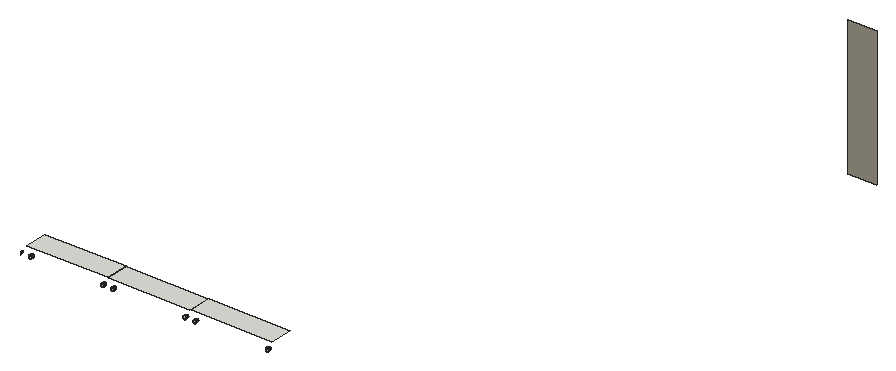
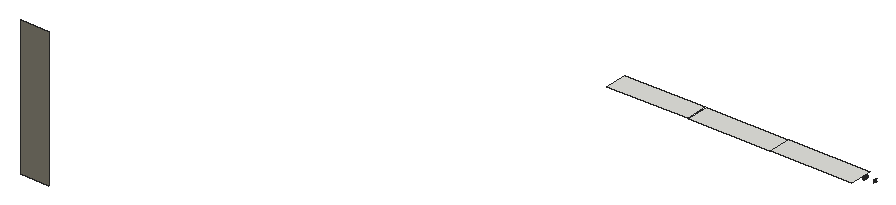
# SketchUp Ruby script. Lengths in inches.
U = 1.inch
M = Sketchup.active_model
def pt(a) = Geom::Point3d.new(a.map { |v| v * U })
def face(e, loops, mat)
  f = e.add_face(loops[0].map { |a| pt(a) })
  loops[1..].each { |l| e.add_face(l.map { |a| pt(a) }).erase! }
  f.material = f.back_material = mat if mat
  f
end
# faces: each face lists its corners as indices into pts; further lists are holes
def faces(e, pts, list, mat = nil) = list.each { |f| face(e, (f[0].is_a?(Array) ? f : [f]).map { |l| l.map { |i| pts[i] } }, mat) }
# xy, xz, yz: faces in a plane at the given z, y or x. An outline is a flat list of corners, or four numbers for a rectangle; further outlines are holes
def ring(l) = l.size == 4 ? [[l[0], l[1]], [l[2], l[1]], [l[2], l[3]], [l[0], l[3]]] : l.each_slice(2).to_a
def flat(e, list, mat, &to3) = list.each { |f| face(e, (f[0].is_a?(Array) ? f : [f]).map { |l| ring(l).map { |u, v| to3.(u, v) } }, mat) }
def xy(e, z, list, mat = nil) = flat(e, list, mat) { |x, y| [x, y, z] }
def xz(e, y, list, mat = nil) = flat(e, list, mat) { |x, z| [x, y, z] }
def yz(e, x, list, mat = nil) = flat(e, list, mat) { |y, z| [x, y, z] }
def lines(e, pts, list) = list.each { |a, b| e.add_line(pt(pts[a]), pt(pts[b])) }
# prism: a flat outline (further loops are holes) pulled along v
def prism(e, loops, v, mat = nil)
  f = face(e, loops, mat); d = Geom::Vector3d.new(v.map { |x| x * U })
  f.pushpull(f.normal.samedirection?(d) ? d.length : -d.length)
end
def box(e, o, s, mat = nil) = prism(e, [[o, [o[0] + s[0], o[1], o[2]], [o[0] + s[0], o[1] + s[1], o[2]], [o[0], o[1] + s[1], o[2]]]], [0, 0, s[2]], mat)
def at(x, y, z, deg = 0) = Geom::Transformation.translation(pt([x, y, z])) * Geom::Transformation.rotation(ORIGIN, Z_AXIS, deg.degrees)
def axes(o, x, y, z) = Geom::Transformation.new([*x, 0, *y, 0, *z, 0, *pt(o).to_a, 1])
def part(name) = M.definitions.add(name)
# library, detail: a bought-in or finely detailed component or shape, given as its bounding box
def library(name, o, s) = part(name).tap { |d| box(d.entities, o, s) }
def detail(e, o, s) = box(e.add_group.entities, o, s)
def put(e, d, t, mat = nil) = e.add_instance(d, t).tap { |i| i.material = mat if mat }
def group(e, t, mat = nil) = e.add_group.tap { |g| g.transformation = t; g.material = mat if mat }.entities
root = M.entities
M.materials.add("[Concrete Tile]").color = [155, 150, 134]
xy(root,138.0625,[[1787.65,801.78,1844.77,817.6],[1845.83,801.78,1902.82,817.6],[1904.13,801.78,1960.87,817.6]])
xz(root,799.91,[[1791.54,131.88,1791.83,131.92,1792.1,132.03,1792.34,132.21,1792.51,132.44,1792.63,132.71,1792.67,133,1792.63,133.29,1792.51,133.57,1792.34,133.8,1792.1,133.98,1791.83,134.09,1791.54,134.13,1791.25,134.09,1790.98,133.98,1790.74,133.8,1790.57,133.57,1790.45,133.29,1790.42,133,1790.45,132.71,1790.57,132.44,1790.74,132.21,1790.98,132.03,1791.25,131.92],[1842.67,131.88,1842.96,131.92,1843.23,132.03,1843.46,132.21,1843.64,132.44,1843.75,132.71,1843.79,133,1843.75,133.29,1843.64,133.57,1843.46,133.8,1843.23,133.98,1842.96,134.09,1842.67,134.13,1842.375,134.09,1842.1,133.98,1841.87,133.8,1841.69,133.57,1841.58,133.29,1841.54,133,1841.58,132.71,1841.69,132.44,1841.87,132.21,1842.1,132.03,1842.375,131.92],[1849.72,131.88,1850.01,131.92,1850.28,132.03,1850.51,132.21,1850.69,132.44,1850.8,132.71,1850.84,133,1850.8,133.29,1850.69,133.57,1850.51,133.8,1850.28,133.98,1850.01,134.09,1849.72,134.13,1849.42,134.09,1849.15,133.98,1848.92,133.8,1848.74,133.57,1848.63,133.29,1848.59,133,1848.63,132.71,1848.74,132.44,1848.92,132.21,1849.15,132.03,1849.42,131.92],[1900.84,131.88,1901.13,131.92,1901.4,132.03,1901.64,132.21,1901.82,132.44,1901.93,132.71,1901.97,133,1901.93,133.29,1901.82,133.57,1901.64,133.8,1901.4,133.98,1901.13,134.09,1900.84,134.13,1900.55,134.09,1900.28,133.98,1900.05,133.8,1899.87,133.57,1899.75,133.29,1899.72,133,1899.75,132.71,1899.87,132.44,1900.05,132.21,1900.28,132.03,1900.55,131.92],[1908.02,131.88,1908.31,131.92,1908.58,132.03,1908.8125,132.21,1908.99,132.44,1909.1,132.71,1909.14,133,1909.1,133.29,1908.99,133.57,1908.8125,133.8,1908.58,133.98,1908.31,134.09,1908.02,134.13,1907.73,134.09,1907.45,133.98,1907.22,133.8,1907.04,133.57,1906.93,133.29,1906.89,133,1906.93,132.71,1907.04,132.44,1907.22,132.21,1907.45,132.03,1907.73,131.92],
  [1959.14,131.88,1959.43,131.92,1959.7,132.03,1959.9375,132.21,1960.12,132.44,1960.23,132.71,1960.27,133,1960.23,133.29,1960.12,133.57,1959.9375,133.8,1959.7,133.98,1959.43,134.09,1959.14,134.13,1958.85,134.09,1958.58,133.98,1958.35,133.8,1958.17,133.57,1958.06,133.29,1958.02,133,1958.06,132.71,1958.17,132.44,1958.35,132.21,1958.58,132.03,1958.85,131.92]])
xz(root,1122.97,[[2112.0625,156.5,2132.1875,254.125]],"[Concrete Tile]")
p = [[1790.98,801.78,132.03],[1791.25,801.78,131.92],[1791.25,799.91,131.92],[1790.98,799.91,132.03],[1791.54,801.78,131.88],[1791.54,799.91,131.88],
  [1791.83,801.78,131.92],[1791.83,799.91,131.92],[1792.1,801.78,132.03],[1792.1,799.91,132.03],[1842.1,801.78,132.03],[1842.375,801.78,131.92],
  [1842.375,799.91,131.92],[1842.1,799.91,132.03],[1842.67,801.78,131.88],[1842.67,799.91,131.88],[1842.96,801.78,131.92],[1842.96,799.91,131.92],
  [1843.23,801.78,132.03],[1843.23,799.91,132.03],[1849.15,801.78,132.03],[1849.42,801.78,131.92],[1849.42,799.91,131.92],[1849.15,799.91,132.03],
  [1849.72,801.78,131.88],[1849.72,799.91,131.88],[1850.01,801.78,131.92],[1850.01,799.91,131.92],[1850.28,801.78,132.03],[1850.28,799.91,132.03],
  [1900.28,801.78,132.03],[1900.55,801.78,131.92],[1900.55,799.91,131.92],[1900.28,799.91,132.03],[1900.84,801.78,131.88],[1900.84,799.91,131.88],
  [1901.13,801.78,131.92],[1901.13,799.91,131.92],[1901.4,801.78,132.03],[1901.4,799.91,132.03],[1907.45,801.78,132.03],[1907.73,801.78,131.92],
  [1907.73,799.91,131.92],[1907.45,799.91,132.03],[1908.02,801.78,131.88],[1908.02,799.91,131.88],[1908.31,801.78,131.92],[1908.31,799.91,131.92],
  [1908.58,801.78,132.03],[1908.58,799.91,132.03],[1958.58,801.78,132.03],[1958.85,801.78,131.92],[1958.85,799.91,131.92],[1958.58,799.91,132.03],
  [1959.14,801.78,131.88],[1959.14,799.91,131.88],[1959.43,801.78,131.92],[1959.43,799.91,131.92],[1959.7,801.78,132.03],[1959.7,799.91,132.03],
  [1790.74,801.78,132.21],[1790.74,799.91,132.21],[1792.34,801.78,132.21],[1792.34,799.91,132.21],[1841.87,801.78,132.21],[1841.87,799.91,132.21],
  [1843.46,801.78,132.21],[1843.46,799.91,132.21],[1848.92,801.78,132.21],[1848.92,799.91,132.21],[1850.51,801.78,132.21],[1850.51,799.91,132.21],
  [1900.05,801.78,132.21],[1900.05,799.91,132.21],[1901.64,801.78,132.21],[1901.64,799.91,132.21],[1907.22,801.78,132.21],[1907.22,799.91,132.21],
  [1908.8125,801.78,132.21],[1908.8125,799.91,132.21],[1958.35,801.78,132.21],[1958.35,799.91,132.21],[1959.9375,801.78,132.21],[1959.9375,799.91,132.21],
  [1784.47,801.78,132.21],[1784.65,801.78,132.44],[1784.65,799.91,132.44],[1784.47,799.91,132.21],[1790.57,801.78,132.44],[1790.57,799.91,132.44],
  [1792.51,801.78,132.44],[1792.51,799.91,132.44],[1841.69,801.78,132.44],[1841.69,799.91,132.44],[1843.64,801.78,132.44],[1843.64,799.91,132.44],
  [1848.74,801.78,132.44],[1848.74,799.91,132.44],[1850.69,801.78,132.44],[1850.69,799.91,132.44],[1899.87,801.78,132.44],[1899.87,799.91,132.44],
  [1901.82,801.78,132.44],[1901.82,799.91,132.44],[1907.04,801.78,132.44],[1907.04,799.91,132.44],[1908.99,801.78,132.44],[1908.99,799.91,132.44],
  [1958.17,801.78,132.44],[1958.17,799.91,132.44],[1960.12,801.78,132.44],[1960.12,799.91,132.44],[1784.76,801.78,132.71],[1784.76,799.91,132.71],
  [1790.45,801.78,132.71],[1790.45,799.91,132.71],[1792.63,801.78,132.71],[1792.63,799.91,132.71],[1841.58,801.78,132.71],[1841.58,799.91,132.71],
  [1843.75,801.78,132.71],[1843.75,799.91,132.71],[1848.63,801.78,132.71],[1848.63,799.91,132.71],[1850.8,801.78,132.71],[1850.8,799.91,132.71],
  [1899.75,801.78,132.71],[1899.75,799.91,132.71],[1901.93,801.78,132.71],[1901.93,799.91,132.71],[1906.93,801.78,132.71],[1906.93,799.91,132.71],
  [1909.1,801.78,132.71],[1909.1,799.91,132.71],[1958.06,801.78,132.71],[1958.06,799.91,132.71],[1960.23,801.78,132.71],[1960.23,799.91,132.71],
  [1784.8,801.78,133],[1784.8,799.91,133],[1790.42,801.78,133],[1790.42,799.91,133],[1792.67,801.78,133],[1792.67,799.91,133],
  [1841.54,801.78,133],[1841.54,799.91,133],[1843.79,801.78,133],[1843.79,799.91,133],[1848.59,801.78,133],[1848.59,799.91,133],
  [1850.84,801.78,133],[1850.84,799.91,133],[1899.72,801.78,133],[1899.72,799.91,133],[1901.97,801.78,133],[1901.97,799.91,133],
  [1906.89,801.78,133],[1906.89,799.91,133],[1909.14,801.78,133],[1909.14,799.91,133],[1958.02,801.78,133],[1958.02,799.91,133],
  [1960.27,801.78,133],[1960.27,799.91,133],[1784.76,801.78,133.29],[1784.76,799.91,133.29],[1790.45,801.78,133.29],[1790.45,799.91,133.29],
  [1792.63,801.78,133.29],[1792.63,799.91,133.29],[1841.58,801.78,133.29],[1841.58,799.91,133.29],[1843.75,801.78,133.29],[1843.75,799.91,133.29],
  [1848.63,801.78,133.29],[1848.63,799.91,133.29],[1850.8,801.78,133.29],[1850.8,799.91,133.29],[1899.75,801.78,133.29],[1899.75,799.91,133.29],
  [1901.93,801.78,133.29],[1901.93,799.91,133.29],[1906.93,801.78,133.29],[1906.93,799.91,133.29],[1909.1,801.78,133.29],[1909.1,799.91,133.29],
  [1958.06,801.78,133.29],[1958.06,799.91,133.29],[1960.23,801.78,133.29],[1960.23,799.91,133.29],[1784.65,801.78,133.57],[1784.65,799.91,133.57],
  [1790.57,801.78,133.57],[1790.57,799.91,133.57],[1792.51,801.78,133.57],[1792.51,799.91,133.57],[1841.69,801.78,133.57],[1841.69,799.91,133.57],
  [1843.64,801.78,133.57],[1843.64,799.91,133.57],[1848.74,801.78,133.57],[1848.74,799.91,133.57],[1850.69,801.78,133.57],[1850.69,799.91,133.57],
  [1899.87,801.78,133.57],[1899.87,799.91,133.57],[1901.82,801.78,133.57],[1901.82,799.91,133.57],[1907.04,801.78,133.57],[1907.04,799.91,133.57],
  [1908.99,801.78,133.57],[1908.99,799.91,133.57],[1958.17,801.78,133.57],[1958.17,799.91,133.57],[1960.12,801.78,133.57],[1960.12,799.91,133.57],
  [1784.47,801.78,133.8],[1784.47,799.91,133.8],[1790.74,801.78,133.8],[1790.74,799.91,133.8],[1792.34,801.78,133.8],[1792.34,799.91,133.8],
  [1841.87,801.78,133.8],[1841.87,799.91,133.8],[1843.46,801.78,133.8],[1843.46,799.91,133.8],[1848.92,801.78,133.8],[1848.92,799.91,133.8],
  [1850.51,801.78,133.8],[1850.51,799.91,133.8],[1900.05,801.78,133.8],[1900.05,799.91,133.8],[1901.64,801.78,133.8],[1901.64,799.91,133.8],
  [1907.22,801.78,133.8],[1907.22,799.91,133.8],[1908.8125,801.78,133.8],[1908.8125,799.91,133.8],[1958.35,801.78,133.8],[1958.35,799.91,133.8],
  [1959.9375,801.78,133.8],[1959.9375,799.91,133.8],[1790.98,801.78,133.98],[1790.98,799.91,133.98],[1792.1,801.78,133.98],[1792.1,799.91,133.98],
  [1842.1,801.78,133.98],[1842.1,799.91,133.98],[1843.23,801.78,133.98],[1843.23,799.91,133.98],[1849.15,801.78,133.98],[1849.15,799.91,133.98],
  [1850.28,801.78,133.98],[1850.28,799.91,133.98],[1900.28,801.78,133.98],[1900.28,799.91,133.98],[1901.4,801.78,133.98],[1901.4,799.91,133.98],
  [1907.45,801.78,133.98],[1907.45,799.91,133.98],[1908.58,801.78,133.98],[1908.58,799.91,133.98],[1958.58,801.78,133.98],[1958.58,799.91,133.98],
  [1959.7,801.78,133.98],[1959.7,799.91,133.98],[1791.25,801.78,134.09],[1791.25,799.91,134.09],[1791.83,801.78,134.09],[1791.83,799.91,134.09],
  [1842.375,801.78,134.09],[1842.375,799.91,134.09],[1842.96,801.78,134.09],[1842.96,799.91,134.09],[1849.42,801.78,134.09],[1849.42,799.91,134.09],
  [1850.01,801.78,134.09],[1850.01,799.91,134.09],[1900.55,801.78,134.09],[1900.55,799.91,134.09],[1901.13,801.78,134.09],[1901.13,799.91,134.09],
  [1907.73,801.78,134.09],[1907.73,799.91,134.09],[1908.31,801.78,134.09],[1908.31,799.91,134.09],[1958.85,801.78,134.09],[1958.85,799.91,134.09],
  [1959.43,801.78,134.09],[1959.43,799.91,134.09],[1791.54,801.78,134.13],[1791.54,799.91,134.13],[1842.67,801.78,134.13],[1842.67,799.91,134.13],
  [1849.72,801.78,134.13],[1849.72,799.91,134.13],[1900.84,801.78,134.13],[1900.84,799.91,134.13],[1908.02,801.78,134.13],[1908.02,799.91,134.13],
  [1959.14,801.78,134.13],[1959.14,799.91,134.13]]
faces(root,p,[[0,1,2,3],[1,4,5,2],[4,6,7,5],[6,8,9,7],[10,11,12,13],[11,14,15,12],[14,16,17,15],[16,18,19,17],
  [20,21,22,23],[21,24,25,22],[24,26,27,25],[26,28,29,27],[30,31,32,33],[31,34,35,32],[34,36,37,35],[36,38,39,37],
  [40,41,42,43],[41,44,45,42],[44,46,47,45],[46,48,49,47],[50,51,52,53],[51,54,55,52],[54,56,57,55],[56,58,59,57],
  [60,0,3,61],[8,62,63,9],[64,10,13,65],[18,66,67,19],[68,20,23,69],[28,70,71,29],[72,30,33,73],[38,74,75,39],
  [76,40,43,77],[48,78,79,49],[80,50,53,81],[58,82,83,59],[84,85,86,87],[88,60,61,89],[62,90,91,63],[92,64,65,93],
  [66,94,95,67],[96,68,69,97],[70,98,99,71],[100,72,73,101],[74,102,103,75],[104,76,77,105],[78,106,107,79],[108,80,81,109],
  [82,110,111,83],[85,112,113,86],[114,88,89,115],[90,116,117,91],[118,92,93,119],[94,120,121,95],[122,96,97,123],[98,124,125,99],
  [126,100,101,127],[102,128,129,103],[130,104,105,131],[106,132,133,107],[134,108,109,135],[110,136,137,111],[112,138,139,113],[140,114,115,141],
  [116,142,143,117],[144,118,119,145],[120,146,147,121],[148,122,123,149],[124,150,151,125],[152,126,127,153],[128,154,155,129],[156,130,131,157],
  [132,158,159,133],[160,134,135,161],[136,162,163,137],[138,164,165,139],[166,140,141,167],[142,168,169,143],[170,144,145,171],[146,172,173,147],
  [174,148,149,175],[150,176,177,151],[178,152,153,179],[154,180,181,155],[182,156,157,183],[158,184,185,159],[186,160,161,187],[162,188,189,163],
  [164,190,191,165],[192,166,167,193],[168,194,195,169],[196,170,171,197],[172,198,199,173],[200,174,175,201],[176,202,203,177],[204,178,179,205],
  [180,206,207,181],[208,182,183,209],[184,210,211,185],[212,186,187,213],[188,214,215,189],[190,216,217,191],[218,192,193,219],[194,220,221,195],
  [222,196,197,223],[198,224,225,199],[226,200,201,227],[202,228,229,203],[230,204,205,231],[206,232,233,207],[234,208,209,235],[210,236,237,211],
  [238,212,213,239],[214,240,241,215],[242,218,219,243],[220,244,245,221],[246,222,223,247],[224,248,249,225],[250,226,227,251],[228,252,253,229],
  [254,230,231,255],[232,256,257,233],[258,234,235,259],[236,260,261,237],[262,238,239,263],[240,264,265,241],[266,242,243,267],[244,268,269,245],
  [270,246,247,271],[248,272,273,249],[274,250,251,275],[252,276,277,253],[278,254,255,279],[256,280,281,257],[282,258,259,283],[260,284,285,261],
  [286,262,263,287],[264,288,289,265],[290,266,267,291],[268,290,291,269],[292,270,271,293],[272,292,293,273],[294,274,275,295],[276,294,295,277],
  [296,278,279,297],[280,296,297,281],[298,282,283,299],[284,298,299,285],[300,286,287,301],[288,300,301,289]])
